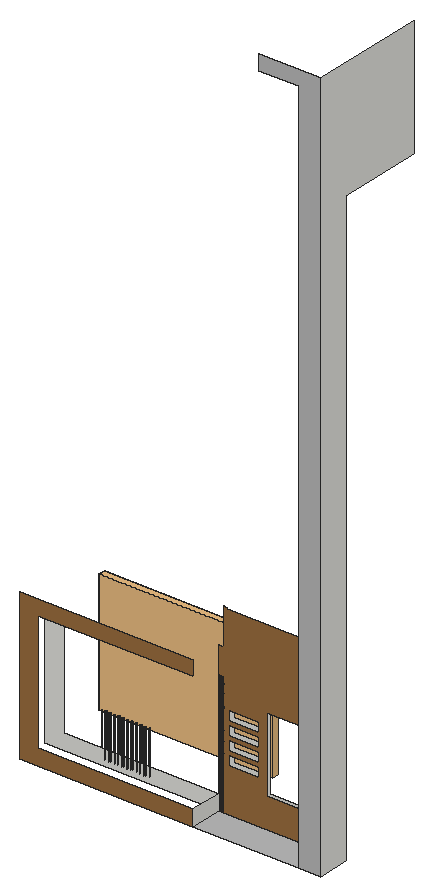
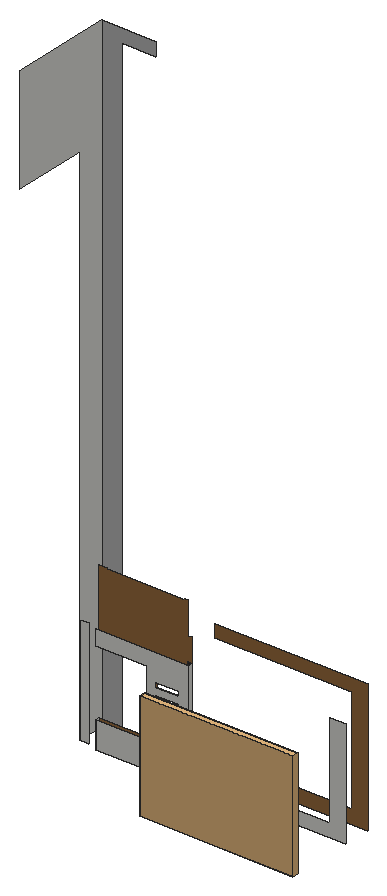
# SketchUp Ruby script. Lengths in inches.
U = 1.inch
M = Sketchup.active_model
def pt(a) = Geom::Point3d.new(a.map { |v| v * U })
def face(e, loops, mat)
  f = e.add_face(loops[0].map { |a| pt(a) })
  loops[1..].each { |l| e.add_face(l.map { |a| pt(a) }).erase! }
  f.material = f.back_material = mat if mat
  f
end
# faces: each face lists its corners as indices into pts; further lists are holes
def faces(e, pts, list, mat = nil) = list.each { |f| face(e, (f[0].is_a?(Array) ? f : [f]).map { |l| l.map { |i| pts[i] } }, mat) }
# xy, xz, yz: faces in a plane at the given z, y or x. An outline is a flat list of corners, or four numbers for a rectangle; further outlines are holes
def ring(l) = l.size == 4 ? [[l[0], l[1]], [l[2], l[1]], [l[2], l[3]], [l[0], l[3]]] : l.each_slice(2).to_a
def flat(e, list, mat, &to3) = list.each { |f| face(e, (f[0].is_a?(Array) ? f : [f]).map { |l| ring(l).map { |u, v| to3.(u, v) } }, mat) }
def xy(e, z, list, mat = nil) = flat(e, list, mat) { |x, y| [x, y, z] }
def xz(e, y, list, mat = nil) = flat(e, list, mat) { |x, z| [x, y, z] }
def yz(e, x, list, mat = nil) = flat(e, list, mat) { |y, z| [x, y, z] }
def lines(e, pts, list) = list.each { |a, b| e.add_line(pt(pts[a]), pt(pts[b])) }
# prism: a flat outline (further loops are holes) pulled along v
def prism(e, loops, v, mat = nil)
  f = face(e, loops, mat); d = Geom::Vector3d.new(v.map { |x| x * U })
  f.pushpull(f.normal.samedirection?(d) ? d.length : -d.length)
end
def box(e, o, s, mat = nil) = prism(e, [[o, [o[0] + s[0], o[1], o[2]], [o[0] + s[0], o[1] + s[1], o[2]], [o[0], o[1] + s[1], o[2]]]], [0, 0, s[2]], mat)
def at(x, y, z, deg = 0) = Geom::Transformation.translation(pt([x, y, z])) * Geom::Transformation.rotation(ORIGIN, Z_AXIS, deg.degrees)
def axes(o, x, y, z) = Geom::Transformation.new([*x, 0, *y, 0, *z, 0, *pt(o).to_a, 1])
def part(name) = M.definitions.add(name)
# library, detail: a bought-in or finely detailed component or shape, given as its bounding box
def library(name, o, s) = part(name).tap { |d| box(d.entities, o, s) }
def detail(e, o, s) = box(e.add_group.entities, o, s)
def put(e, d, t, mat = nil) = e.add_instance(d, t).tap { |i| i.material = mat if mat }
def group(e, t, mat = nil) = e.add_group.tap { |g| g.transformation = t; g.material = mat if mat }.entities
root = M.entities
M.materials.add("Generic").color = [155, 110, 63]
M.materials.add("Generic\#2").color = [186, 186, 186]
M.materials.add("Generic\#4").color = [48, 45, 45]
c1 = library("Group\#9",[0,0,0],[238.3125,8.75,168])
xy(root,204.9375,[[528.75,124.5,673.48,130.75]])
xy(root,204.9375,[[528.75,81.125,673.48,124.5]],"Generic\#2")
xz(root,81.125,[[290.4375,204.9375,528.75,204.9375,528.75,226.375,315.5625,226.375,315.5625,390.1875,528.75,390.1875,528.75,409.875,290.4375,409.875]],"Generic")
xz(root,81.125,[[673.48,204.9375,703.6875,204.9375,703.6875,1189.3125,619.48,1189.3125,619.48,1168.125,673.48,1168.125]],"Generic\#2")
xz(root,124.5,[[290.4375,204.9375,290.4375,372.9375,315.5625,372.9375,315.5625,226.375,528.75,226.375,528.75,204.9375],[690.4375,204.9375,703.6875,372.9375]])
xz(root,124.5,[[[535.75,204.9375,673.48,204.9375,673.48,246.29,594.67,246.29,594.67,349.35,673.48,349.35,673.48,459.625,662.53,459.625,662.53,458.4,540.25,458.4,540.25,459.625,535.75,459.625,535.75,409.875,528.75,409.875,528.75,372.9375,535.75,372.9375],[542.55,320.57,583.96,334.54],[542.55,302.07,583.96,316.04],[542.55,283.57,583.96,297.54],[542.55,265.07,583.96,279.04]]],"Generic")
xz(root,124.5,[[528.75,204.9375,535.75,372.9375]],"Generic\#4")
xz(root,130.75,[[[528.75,204.9375,528.75,372.9375,673.48,372.9375,673.48,349.35,594.67,349.35,594.67,246.29,673.48,246.29,673.48,204.9375],[545.16,267.68,581.35,276.43],[545.16,286.18,581.35,294.93],[545.16,304.68,581.35,313.43],[545.16,323.18,581.35,331.93]]])
yz(root,528.75,[[81.125,204.9375,124.5,226.375],[124.5,204.9375,130.75,372.9375]])
yz(root,673.48,[[124.5,204.9375,130.75,246.29]])
yz(root,703.6875,[[81.125,204.9375,124.5,204.9375,124.5,1024.6875,241.25,1024.6875,241.25,1189.3125,81.125,1189.3125]])
p = [[363.86,135.42,204.9375],[364.06,135.34,204.9375],[364.06,135.34,264.83],[363.86,135.42,264.83],[364.27,135.31,204.9375],[364.27,135.31,264.83],
  [364.48,135.34,204.9375],[364.48,135.34,264.83],[364.67,135.42,204.9375],[364.67,135.42,264.83],[369.8,135.42,204.9375],[369.99,135.34,204.9375],
  [369.99,135.34,264.83],[369.8,135.42,264.83],[370.2,135.31,204.9375],[370.2,135.31,264.83],[370.41,135.34,204.9375],[370.41,135.34,264.83],
  [370.61,135.42,204.9375],[370.61,135.42,264.83],[375.86,135.42,204.9375],[376.06,135.34,204.9375],[376.06,135.34,264.83],[375.86,135.42,264.83],
  [376.27,135.31,204.9375],[376.27,135.31,264.83],[376.48,135.34,204.9375],[376.48,135.34,264.83],[376.67,135.42,204.9375],[376.67,135.42,264.83],
  [381.86,135.42,204.9375],[382.06,135.34,204.9375],[382.06,135.34,264.83],[381.86,135.42,264.83],[382.27,135.31,204.9375],[382.27,135.31,264.83],
  [382.48,135.34,204.9375],[382.48,135.34,264.83],[382.67,135.42,204.9375],[382.67,135.42,264.83],[387.67,135.42,204.9375],[387.87,135.34,204.9375],
  [387.87,135.34,264.83],[387.67,135.42,264.83],[388.08,135.31,204.9375],[388.08,135.31,264.83],[388.29,135.34,204.9375],[388.29,135.34,264.83],
  [388.49,135.42,204.9375],[388.49,135.42,264.83],[393.8,135.42,204.9375],[393.99,135.34,204.9375],[393.99,135.34,264.83],[393.8,135.42,264.83],
  [394.2,135.31,204.9375],[394.2,135.31,264.83],[394.41,135.34,204.9375],[394.41,135.34,264.83],[394.61,135.42,204.9375],[394.61,135.42,264.83],
  [399.92,135.42,204.9375],[400.12,135.34,204.9375],[400.12,135.34,264.83],[399.92,135.42,264.83],[400.33,135.31,204.9375],[400.33,135.31,264.83],
  [400.54,135.34,204.9375],[400.54,135.34,264.83],[400.74,135.42,204.9375],[400.74,135.42,264.83],[405.92,135.42,204.9375],[406.12,135.34,204.9375],
  [406.12,135.34,264.83],[405.92,135.42,264.83],[406.33,135.31,204.9375],[406.33,135.31,264.83],[406.54,135.34,204.9375],[406.54,135.34,264.83],
  [406.74,135.42,204.9375],[406.74,135.42,264.83],[411.92,135.42,204.9375],[412.12,135.34,204.9375],[412.12,135.34,264.83],[411.92,135.42,264.83],
  [412.33,135.31,204.9375],[412.33,135.31,264.83],[412.54,135.34,204.9375],[412.54,135.34,264.83],[412.74,135.42,204.9375],[412.74,135.42,264.83],
  [417.92,135.42,204.9375],[418.12,135.34,204.9375],[418.12,135.34,264.83],[417.92,135.42,264.83],[418.33,135.31,204.9375],[418.33,135.31,264.83],
  [418.54,135.34,204.9375],[418.54,135.34,264.83],[418.74,135.42,204.9375],[418.74,135.42,264.83],[423.92,135.42,204.9375],[424.12,135.34,204.9375],
  [424.12,135.34,264.83],[423.92,135.42,264.83],[424.33,135.31,204.9375],[424.33,135.31,264.83],[424.54,135.34,204.9375],[424.54,135.34,264.83],
  [424.74,135.42,204.9375],[424.74,135.42,264.83],[363.69,135.55,204.9375],[363.69,135.55,264.83],[364.84,135.55,204.9375],[364.84,135.55,264.83],
  [369.63,135.55,204.9375],[369.63,135.55,264.83],[370.78,135.55,204.9375],[370.78,135.55,264.83],[375.69,135.55,204.9375],[375.69,135.55,264.83],
  [376.84,135.55,204.9375],[376.84,135.55,264.83],[381.69,135.55,204.9375],[381.69,135.55,264.83],[382.84,135.55,204.9375],[382.84,135.55,264.83],
  [387.5,135.55,204.9375],[387.5,135.55,264.83],[388.65,135.55,204.9375],[388.65,135.55,264.83],[393.63,135.55,204.9375],[393.63,135.55,264.83],
  [394.78,135.55,204.9375],[394.78,135.55,264.83],[399.75,135.55,204.9375],[399.75,135.55,264.83],[400.9,135.55,204.9375],[400.9,135.55,264.83],
  [405.75,135.55,204.9375],[405.75,135.55,264.83],[406.9,135.55,204.9375],[406.9,135.55,264.83],[411.75,135.55,204.9375],[411.75,135.55,264.83],
  [412.9,135.55,204.9375],[412.9,135.55,264.83],[417.75,135.55,204.9375],[417.75,135.55,264.83],[418.9,135.55,204.9375],[418.9,135.55,264.83],
  [423.75,135.55,204.9375],[423.75,135.55,264.83],[424.9,135.55,204.9375],[424.9,135.55,264.83],[358.84,135.55,204.9375],[358.97,135.72,204.9375],
  [358.97,135.72,264.83],[358.84,135.55,264.83],[363.5625,135.72,204.9375],[363.5625,135.72,264.83],[364.97,135.72,204.9375],[364.97,135.72,264.83],
  [369.5,135.72,204.9375],[369.5,135.72,264.83],[370.91,135.72,204.9375],[370.91,135.72,264.83],[375.5625,135.72,204.9375],[375.5625,135.72,264.83],
  [376.97,135.72,204.9375],[376.97,135.72,264.83],[381.5625,135.72,204.9375],[381.5625,135.72,264.83],[382.97,135.72,204.9375],[382.97,135.72,264.83],
  [387.375,135.72,204.9375],[387.375,135.72,264.83],[388.78,135.72,204.9375],[388.78,135.72,264.83],[393.5,135.72,204.9375],[393.5,135.72,264.83],
  [394.91,135.72,204.9375],[394.91,135.72,264.83],[399.625,135.72,204.9375],[399.625,135.72,264.83],[401.03,135.72,204.9375],[401.03,135.72,264.83],
  [405.625,135.72,204.9375],[405.625,135.72,264.83],[407.03,135.72,204.9375],[407.03,135.72,264.83],[411.625,135.72,204.9375],[411.625,135.72,264.83],
  [413.03,135.72,204.9375],[413.03,135.72,264.83],[417.625,135.72,204.9375],[417.625,135.72,264.83],[419.03,135.72,204.9375],[419.03,135.72,264.83],
  [423.625,135.72,204.9375],[423.625,135.72,264.83],[425.03,135.72,204.9375],[425.03,135.72,264.83],[359.05,135.91,204.9375],[359.05,135.91,264.83],
  [363.48,135.91,204.9375],[363.48,135.91,264.83],[365.05,135.91,204.9375],[365.05,135.91,264.83],[369.42,135.91,204.9375],[369.42,135.91,264.83],
  [370.99,135.91,204.9375],[370.99,135.91,264.83],[375.48,135.91,204.9375],[375.48,135.91,264.83],[377.05,135.91,204.9375],[377.05,135.91,264.83],
  [381.48,135.91,204.9375],[381.48,135.91,264.83],[383.05,135.91,204.9375],[383.05,135.91,264.83],[387.29,135.91,204.9375],[387.29,135.91,264.83],
  [388.86,135.91,204.9375],[388.86,135.91,264.83],[393.42,135.91,204.9375],[393.42,135.91,264.83],[394.99,135.91,204.9375],[394.99,135.91,264.83],
  [399.54,135.91,204.9375],[399.54,135.91,264.83],[401.11,135.91,204.9375],[401.11,135.91,264.83],[405.54,135.91,204.9375],[405.54,135.91,264.83],
  [407.11,135.91,204.9375],[407.11,135.91,264.83],[411.54,135.91,204.9375],[411.54,135.91,264.83],[413.11,135.91,204.9375],[413.11,135.91,264.83],
  [417.54,135.91,204.9375],[417.54,135.91,264.83],[419.11,135.91,204.9375],[419.11,135.91,264.83],[423.54,135.91,204.9375],[423.54,135.91,264.83],
  [425.11,135.91,204.9375],[425.11,135.91,264.83],[359.08,136.12,204.9375],[359.08,136.12,264.83],[363.45,136.12,204.9375],[363.45,136.12,264.83],
  [365.08,136.12,204.9375],[365.08,136.12,264.83],[369.39,136.12,204.9375],[369.39,136.12,264.83],[371.02,136.12,204.9375],[371.02,136.12,264.83],
  [375.45,136.12,204.9375],[375.45,136.12,264.83],[377.08,136.12,204.9375],[377.08,136.12,264.83],[381.45,136.12,204.9375],[381.45,136.12,264.83],
  [383.08,136.12,204.9375],[383.08,136.12,264.83],[387.27,136.12,204.9375],[387.27,136.12,264.83],[388.89,136.12,204.9375],[388.89,136.12,264.83],
  [393.39,136.12,204.9375],[393.39,136.12,264.83],[395.02,136.12,204.9375],[395.02,136.12,264.83],[399.52,136.12,204.9375],[399.52,136.12,264.83],
  [401.14,136.12,204.9375],[401.14,136.12,264.83],[405.52,136.12,204.9375],[405.52,136.12,264.83],[407.14,136.12,204.9375],[407.14,136.12,264.83],
  [411.52,136.12,204.9375],[411.52,136.12,264.83],[413.14,136.12,204.9375],[413.14,136.12,264.83],[417.52,136.12,204.9375],[417.52,136.12,264.83],
  [419.14,136.12,204.9375],[419.14,136.12,264.83],[425.14,136.12,204.9375],[425.14,136.12,264.83],[359.05,136.33,204.9375],[359.05,136.33,264.83],
  [363.48,136.33,204.9375],[363.48,136.33,264.83],[365.05,136.33,204.9375],[365.05,136.33,264.83],[369.42,136.33,204.9375],[369.42,136.33,264.83],
  [370.99,136.33,204.9375],[370.99,136.33,264.83],[375.48,136.33,204.9375],[375.48,136.33,264.83],[377.05,136.33,204.9375],[377.05,136.33,264.83],
  [381.48,136.33,204.9375],[381.48,136.33,264.83],[383.05,136.33,204.9375],[383.05,136.33,264.83],[387.29,136.33,204.9375],[387.29,136.33,264.83],
  [388.86,136.33,204.9375],[388.86,136.33,264.83],[393.42,136.33,204.9375],[393.42,136.33,264.83],[394.99,136.33,204.9375],[394.99,136.33,264.83],
  [399.54,136.33,204.9375],[399.54,136.33,264.83],[401.11,136.33,204.9375],[401.11,136.33,264.83],[405.54,136.33,204.9375],[405.54,136.33,264.83],
  [407.11,136.33,204.9375],[407.11,136.33,264.83],[411.54,136.33,204.9375],[411.54,136.33,264.83],[413.11,136.33,204.9375],[413.11,136.33,264.83],
  [417.54,136.33,204.9375],[417.54,136.33,264.83],[419.11,136.33,204.9375],[419.11,136.33,264.83],[425.11,136.33,204.9375],[425.11,136.33,264.83],
  [358.97,136.53,204.9375],[358.97,136.53,264.83],[363.5625,136.53,204.9375],[363.5625,136.53,264.83],[364.97,136.53,204.9375],[364.97,136.53,264.83],
  [369.5,136.53,204.9375],[369.5,136.53,264.83],[370.91,136.53,204.9375],[370.91,136.53,264.83],[375.5625,136.53,204.9375],[375.5625,136.53,264.83],
  [376.97,136.53,204.9375],[376.97,136.53,264.83],[381.5625,136.53,204.9375],[381.5625,136.53,264.83],[382.97,136.53,204.9375],[382.97,136.53,264.83],
  [387.375,136.53,204.9375],[387.375,136.53,264.83],[388.78,136.53,204.9375],[388.78,136.53,264.83],[393.5,136.53,204.9375],[393.5,136.53,264.83],
  [394.91,136.53,204.9375],[394.91,136.53,264.83],[399.625,136.53,204.9375],[399.625,136.53,264.83],[401.03,136.53,204.9375],[401.03,136.53,264.83],
  [405.625,136.53,204.9375],[405.625,136.53,264.83],[407.03,136.53,204.9375],[407.03,136.53,264.83],[411.625,136.53,204.9375],[411.625,136.53,264.83],
  [413.03,136.53,204.9375],[413.03,136.53,264.83],[417.625,136.53,204.9375],[417.625,136.53,264.83],[419.03,136.53,204.9375],[419.03,136.53,264.83],
  [425.03,136.53,204.9375],[425.03,136.53,264.83],[363.69,136.7,204.9375],[363.69,136.7,264.83],[364.84,136.7,204.9375],[364.84,136.7,264.83],
  [369.63,136.7,204.9375],[369.63,136.7,264.83],[370.78,136.7,204.9375],[370.78,136.7,264.83],[375.69,136.7,204.9375],[375.69,136.7,264.83],
  [376.84,136.7,204.9375],[376.84,136.7,264.83],[381.69,136.7,204.9375],[381.69,136.7,264.83],[382.84,136.7,204.9375],[382.84,136.7,264.83],
  [387.5,136.7,204.9375],[387.5,136.7,264.83],[388.65,136.7,204.9375],[388.65,136.7,264.83],[393.63,136.7,204.9375],[393.63,136.7,264.83],
  [394.78,136.7,204.9375],[394.78,136.7,264.83],[399.75,136.7,204.9375],[399.75,136.7,264.83],[400.9,136.7,204.9375],[400.9,136.7,264.83],
  [405.75,136.7,204.9375],[405.75,136.7,264.83],[406.9,136.7,204.9375],[406.9,136.7,264.83],[411.75,136.7,204.9375],[411.75,136.7,264.83],
  [412.9,136.7,204.9375],[412.9,136.7,264.83],[417.75,136.7,204.9375],[417.75,136.7,264.83],[418.9,136.7,204.9375],[418.9,136.7,264.83],
  [424.9,136.7,204.9375],[424.9,136.7,264.83],[363.86,136.83,204.9375],[363.86,136.83,264.83],[364.67,136.83,204.9375],[364.67,136.83,264.83],
  [369.8,136.83,204.9375],[369.8,136.83,264.83],[370.61,136.83,204.9375],[370.61,136.83,264.83],[375.86,136.83,204.9375],[375.86,136.83,264.83],
  [376.67,136.83,204.9375],[376.67,136.83,264.83],[381.86,136.83,204.9375],[381.86,136.83,264.83],[382.67,136.83,204.9375],[382.67,136.83,264.83],
  [387.67,136.83,204.9375],[387.67,136.83,264.83],[388.49,136.83,204.9375],[388.49,136.83,264.83],[393.8,136.83,204.9375],[393.8,136.83,264.83],
  [394.61,136.83,204.9375],[394.61,136.83,264.83],[399.92,136.83,204.9375],[399.92,136.83,264.83],[400.74,136.83,204.9375],[400.74,136.83,264.83],
  [405.92,136.83,204.9375],[405.92,136.83,264.83],[406.74,136.83,204.9375],[406.74,136.83,264.83],[411.92,136.83,204.9375],[411.92,136.83,264.83],
  [412.74,136.83,204.9375],[412.74,136.83,264.83],[417.92,136.83,204.9375],[417.92,136.83,264.83],[418.74,136.83,204.9375],[418.74,136.83,264.83],
  [424.74,136.83,204.9375],[424.74,136.83,264.83],[364.06,136.91,204.9375],[364.06,136.91,264.83],[364.48,136.91,204.9375],[364.48,136.91,264.83],
  [369.99,136.91,204.9375],[369.99,136.91,264.83],[370.41,136.91,204.9375],[370.41,136.91,264.83],[376.06,136.91,204.9375],[376.06,136.91,264.83],
  [376.48,136.91,204.9375],[376.48,136.91,264.83],[382.06,136.91,204.9375],[382.06,136.91,264.83],[382.48,136.91,204.9375],[382.48,136.91,264.83],
  [387.87,136.91,204.9375],[387.87,136.91,264.83],[388.29,136.91,204.9375],[388.29,136.91,264.83],[393.99,136.91,204.9375],[393.99,136.91,264.83],
  [394.41,136.91,204.9375],[394.41,136.91,264.83],[400.12,136.91,204.9375],[400.12,136.91,264.83],[400.54,136.91,204.9375],[400.54,136.91,264.83],
  [406.12,136.91,204.9375],[406.12,136.91,264.83],[406.54,136.91,204.9375],[406.54,136.91,264.83],[412.12,136.91,204.9375],[412.12,136.91,264.83],
  [412.54,136.91,204.9375],[412.54,136.91,264.83],[418.12,136.91,204.9375],[418.12,136.91,264.83],[418.54,136.91,204.9375],[418.54,136.91,264.83],
  [424.54,136.91,204.9375],[424.54,136.91,264.83],[364.27,136.93,204.9375],[364.27,136.93,264.83],[370.2,136.93,204.9375],[370.2,136.93,264.83],
  [376.27,136.93,204.9375],[376.27,136.93,264.83],[382.27,136.93,204.9375],[382.27,136.93,264.83],[388.08,136.93,204.9375],[388.08,136.93,264.83],
  [394.2,136.93,204.9375],[394.2,136.93,264.83],[400.33,136.93,204.9375],[400.33,136.93,264.83],[406.33,136.93,204.9375],[406.33,136.93,264.83],
  [412.33,136.93,204.9375],[412.33,136.93,264.83],[418.33,136.93,204.9375],[418.33,136.93,264.83]]
faces(root,p,[[0,1,2,3],[1,4,5,2],[4,6,7,5],[6,8,9,7],[10,11,12,13],[11,14,15,12],[14,16,17,15],[16,18,19,17],
  [20,21,22,23],[21,24,25,22],[24,26,27,25],[26,28,29,27],[30,31,32,33],[31,34,35,32],[34,36,37,35],[36,38,39,37],
  [40,41,42,43],[41,44,45,42],[44,46,47,45],[46,48,49,47],[50,51,52,53],[51,54,55,52],[54,56,57,55],[56,58,59,57],
  [60,61,62,63],[61,64,65,62],[64,66,67,65],[66,68,69,67],[70,71,72,73],[71,74,75,72],[74,76,77,75],[76,78,79,77],
  [80,81,82,83],[81,84,85,82],[84,86,87,85],[86,88,89,87],[90,91,92,93],[91,94,95,92],[94,96,97,95],[96,98,99,97],
  [100,101,102,103],[101,104,105,102],[104,106,107,105],[106,108,109,107],[110,0,3,111],[8,112,113,9],[114,10,13,115],[18,116,117,19],
  [118,20,23,119],[28,120,121,29],[122,30,33,123],[38,124,125,39],[126,40,43,127],[48,128,129,49],[130,50,53,131],[58,132,133,59],
  [134,60,63,135],[68,136,137,69],[138,70,73,139],[78,140,141,79],[142,80,83,143],[88,144,145,89],[146,90,93,147],[98,148,149,99],
  [150,100,103,151],[108,152,153,109],[154,155,156,157],[158,110,111,159],[112,160,161,113],[162,114,115,163],[116,164,165,117],[166,118,119,167],
  [120,168,169,121],[170,122,123,171],[124,172,173,125],[174,126,127,175],[128,176,177,129],[178,130,131,179],[132,180,181,133],[182,134,135,183],
  [136,184,185,137],[186,138,139,187],[140,188,189,141],[190,142,143,191],[144,192,193,145],[194,146,147,195],[148,196,197,149],[198,150,151,199],
  [152,200,201,153],[155,202,203,156],[204,158,159,205],[160,206,207,161],[208,162,163,209],[164,210,211,165],[212,166,167,213],[168,214,215,169],
  [216,170,171,217],[172,218,219,173],[220,174,175,221],[176,222,223,177],[224,178,179,225],[180,226,227,181],[228,182,183,229],[184,230,231,185],
  [232,186,187,233],[188,234,235,189],[236,190,191,237],[192,238,239,193],[240,194,195,241],[196,242,243,197],[244,198,199,245],[200,246,247,201],
  [202,248,249,203],[250,204,205,251],[206,252,253,207],[254,208,209,255],[210,256,257,211],[258,212,213,259],[214,260,261,215],[262,216,217,263],
  [218,264,265,219],[266,220,221,267],[222,268,269,223],[270,224,225,271],[226,272,273,227],[274,228,229,275],[230,276,277,231],[278,232,233,279],
  [234,280,281,235],[282,236,237,283],[238,284,285,239],[286,240,241,287],[242,288,289,243],[246,290,291,247],[248,292,293,249],[294,250,251,295],
  [252,296,297,253],[298,254,255,299],[256,300,301,257],[302,258,259,303],[260,304,305,261],[306,262,263,307],[264,308,309,265],[310,266,267,311],
  [268,312,313,269],[314,270,271,315],[272,316,317,273],[318,274,275,319],[276,320,321,277],[322,278,279,323],[280,324,325,281],[326,282,283,327],
  [284,328,329,285],[330,286,287,331],[288,332,333,289],[290,334,335,291],[292,336,337,293],[338,294,295,339],[296,340,341,297],[342,298,299,343],
  [300,344,345,301],[346,302,303,347],[304,348,349,305],[350,306,307,351],[308,352,353,309],[354,310,311,355],[312,356,357,313],[358,314,315,359],
  [316,360,361,317],[362,318,319,363],[320,364,365,321],[366,322,323,367],[324,368,369,325],[370,326,327,371],[328,372,373,329],[374,330,331,375],
  [332,376,377,333],[334,378,379,335],[380,338,339,381],[340,382,383,341],[384,342,343,385],[344,386,387,345],[388,346,347,389],[348,390,391,349],
  [392,350,351,393],[352,394,395,353],[396,354,355,397],[356,398,399,357],[400,358,359,401],[360,402,403,361],[404,362,363,405],[364,406,407,365],
  [408,366,367,409],[368,410,411,369],[412,370,371,413],[372,414,415,373],[416,374,375,417],[376,418,419,377],[378,420,421,379],[422,380,381,423],
  [382,424,425,383],[426,384,385,427],[386,428,429,387],[430,388,389,431],[390,432,433,391],[434,392,393,435],[394,436,437,395],[438,396,397,439],
  [398,440,441,399],[442,400,401,443],[402,444,445,403],[446,404,405,447],[406,448,449,407],[450,408,409,451],[410,452,453,411],[454,412,413,455],
  [414,456,457,415],[458,416,417,459],[418,460,461,419],[420,462,463,421],[464,422,423,465],[424,466,467,425],[468,426,427,469],[428,470,471,429],
  [472,430,431,473],[432,474,475,433],[476,434,435,477],[436,478,479,437],[480,438,439,481],[440,482,483,441],[484,442,443,485],[444,486,487,445],
  [488,446,447,489],[448,490,491,449],[492,450,451,493],[452,494,495,453],[496,454,455,497],[456,498,499,457],[500,458,459,501],[460,502,503,461],
  [462,504,505,463],[506,464,465,507],[466,506,507,467],[508,468,469,509],[470,508,509,471],[510,472,473,511],[474,510,511,475],[512,476,477,513],
  [478,512,513,479],[514,480,481,515],[482,514,515,483],[516,484,485,517],[486,516,517,487],[518,488,489,519],[490,518,519,491],[520,492,493,521],
  [494,520,521,495],[522,496,497,523],[498,522,523,499],[524,500,501,525],[502,524,525,503]])
put(root,c1,at(290.4375,217.375,204.9375))
